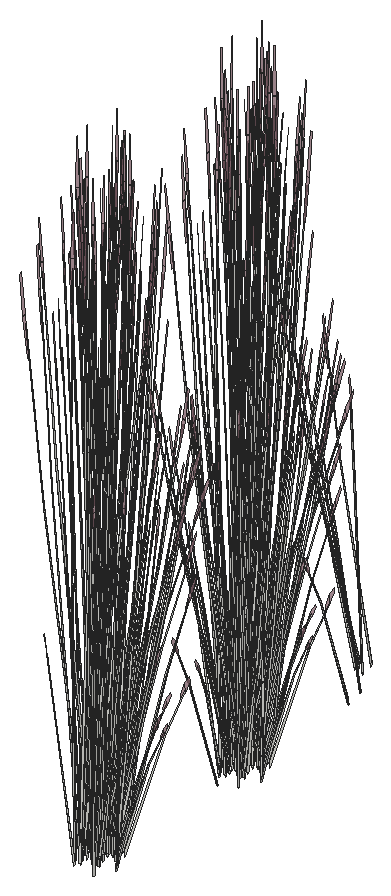
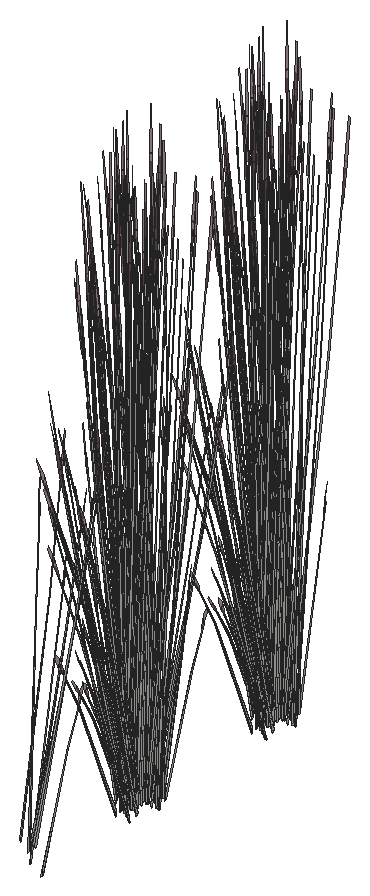
# SketchUp Ruby script. Lengths in inches.
U = 1.inch
M = Sketchup.active_model
def pt(a) = Geom::Point3d.new(a.map { |v| v * U })
def face(e, loops, mat)
  f = e.add_face(loops[0].map { |a| pt(a) })
  loops[1..].each { |l| e.add_face(l.map { |a| pt(a) }).erase! }
  f.material = f.back_material = mat if mat
  f
end
# faces: each face lists its corners as indices into pts; further lists are holes
def faces(e, pts, list, mat = nil) = list.each { |f| face(e, (f[0].is_a?(Array) ? f : [f]).map { |l| l.map { |i| pts[i] } }, mat) }
# xy, xz, yz: faces in a plane at the given z, y or x. An outline is a flat list of corners, or four numbers for a rectangle; further outlines are holes
def ring(l) = l.size == 4 ? [[l[0], l[1]], [l[2], l[1]], [l[2], l[3]], [l[0], l[3]]] : l.each_slice(2).to_a
def flat(e, list, mat, &to3) = list.each { |f| face(e, (f[0].is_a?(Array) ? f : [f]).map { |l| ring(l).map { |u, v| to3.(u, v) } }, mat) }
def xy(e, z, list, mat = nil) = flat(e, list, mat) { |x, y| [x, y, z] }
def xz(e, y, list, mat = nil) = flat(e, list, mat) { |x, z| [x, y, z] }
def yz(e, x, list, mat = nil) = flat(e, list, mat) { |y, z| [x, y, z] }
def lines(e, pts, list) = list.each { |a, b| e.add_line(pt(pts[a]), pt(pts[b])) }
# prism: a flat outline (further loops are holes) pulled along v
def prism(e, loops, v, mat = nil)
  f = face(e, loops, mat); d = Geom::Vector3d.new(v.map { |x| x * U })
  f.pushpull(f.normal.samedirection?(d) ? d.length : -d.length)
end
def box(e, o, s, mat = nil) = prism(e, [[o, [o[0] + s[0], o[1], o[2]], [o[0] + s[0], o[1] + s[1], o[2]], [o[0], o[1] + s[1], o[2]]]], [0, 0, s[2]], mat)
def at(x, y, z, deg = 0) = Geom::Transformation.translation(pt([x, y, z])) * Geom::Transformation.rotation(ORIGIN, Z_AXIS, deg.degrees)
def axes(o, x, y, z) = Geom::Transformation.new([*x, 0, *y, 0, *z, 0, *pt(o).to_a, 1])
def part(name) = M.definitions.add(name)
# library, detail: a bought-in or finely detailed component or shape, given as its bounding box
def library(name, o, s) = part(name).tap { |d| box(d.entities, o, s) }
def detail(e, o, s) = box(e.add_group.entities, o, s)
def put(e, d, t, mat = nil) = e.add_instance(d, t).tap { |i| i.material = mat if mat }
def group(e, t, mat = nil) = e.add_group.tap { |g| g.transformation = t; g.material = mat if mat }.entities
root = M.entities
M.materials.add("LightPink_Translucent").color = [144, 107, 117]
M.materials["LightPink_Translucent"].alpha = 0.75
c1 = part("blade")
p = [[2.15,0.21,22],[0,0.17,0],[0.09,0.45,0],[2.18,0.31,22],[2.29,0.31,22],[0.38,0.45,0],
  [2.48,0.24,33],[2.49,0.24,33],[2.48,0.22,33]]
faces(c1.entities,p,[[0,1,2,3],[4,5,2,3],[6,3,4,7],[8,0,3,6]])
c2 = part("seeds")
p = [[0.3,-0.1,1.38],[-0.01,-0.03,1.59],[-0.01,-0.03,0.03],[0.14,-0.07,-0.07],[0.29,-0.03,3],[0.15,0.01,3.11]]
faces(c2.entities,p,[[0,1,2,3],[1,0,4,5]],"LightPink_Translucent")
c3 = part("blade with seeds")
put(c3.entities,c1,at(0,0,0))
put(c3.entities,c2,axes([2.4,0.25,30.99],[1.5799,-0.05474,1.17369],[-0.12525,1.92788,0.29478],[-0.07173,-0.02425,1.56792]))
put(root,c3,axes([401.49,690.17,2.1],[-0.14494,-0.47823,-0.69835],[0.41752,-0.17223,-0.18329],[-0.01602,-0.16194,1.54149]))
put(root,c3,axes([403.43,688.71,1.49],[-0.05283,-0.03674,1.76342],[-0.13569,-0.41045,-0.26939],[0.09154,-0.11138,0.30037]))
put(root,c3,axes([403.42,689.87,4.98],[0.18436,-0.36797,-0.71045],[0.32306,0.26151,0.08574],[0.11008,-0.13332,1.00501]))
put(root,c3,axes([401.43,688.8,2.375],[-0.22066,-0.46731,0],[0.36918,-0.26061,-0.51607],[0.08408,-0.05936,1.63711]))
put(root,c3,axes([403.41,689.7,4.68],[-0.09067,-0.42583,-0.51099],[0.34336,-0.07449,-0.3958],[0.0984,-0.11438,0.97773]))
put(root,c3,axes([401.92,688.24,2.13],[-0.2439,0.26754,-0.03893],[-0.22348,-0.29302,-0.17649],[-0.01573,-0.08303,0.58215]))
put(root,c3,axes([400.63,690.11,2.02],[0,-0.46636,-0.49651],[0.39487,0,0],[0,-0.10622,1.57504]))
put(root,c3,axes([401.73,688.73,2.02],[0.33032,-0.23318,-0.49651],[0.19744,0.41812,0],[0.07523,-0.05311,1.57504]))
put(root,c3,axes([403.69,689.53,2.59],[-0.12609,-0.01381,1.43002],[-0.12917,-0.37055,-0.30754],[0.1549,-0.10482,0.61141]))
put(root,c3,axes([402.12,689.68,2.06],[0.23773,-0.35053,-0.62353],[0.29532,0.31785,-0.16365],[0.09526,-0.08744,1.37633]))
put(root,c3,axes([403.84,688.85,2.77],[-0.11756,0.2374,1.1486],[-0.10105,-0.31895,0.84392],[0.09709,-0.07992,0.25299]))
put(root,c3,axes([403.67,689.74,4.53],[0.30722,-0.06665,-0.35414],[0.08112,0.381,0.4572],[0.08804,-0.10234,0.87481]))
put(root,c3,axes([401.71,690.3,2.21],[0.17124,-0.42022,-0.44739],[0.35581,0.20224,0.21531],[0,-0.09687,1.43643]))
put(root,c3,axes([401.86,690.09,2.67],[-0.04113,-0.53214,-0.29095],[0.42835,-0.03218,-0.50002],[0.07543,-0.07088,1.59708]))
put(root,c3,axes([400.8,690.12,2.03],[0.24637,-0.29097,-0.30978],[0.24637,0.29097,0.30978],[0,-0.09372,1.38974]))
put(root,c3,axes([401.67,690.65,2.67],[-0.39748,-0.22252,-0.29095],[0.19139,-0.46966,-0.50002],[-0.01249,-0.11531,1.59708]))
put(root,c3,axes([401.81,688.91,2.03],[0.32928,0.11539,-0.30978],[-0.08291,0.40636,0.30978],[0.06638,-0.04686,1.38974]))
put(root,c3,axes([401.92,690.51,2.43],[0.39767,0.22603,0.24065],[-0.19139,0.46966,0.50002],[0,-0.10827,1.60543]))
put(root,c3,axes([401.79,690.19,2.72],[-0.38326,0.02879,0.44739],[-0.03466,-0.47788,-0.21531],[0.06861,-0.04843,1.43643]))
put(root,c3,axes([400.8,690.54,2.48],[0,0.46636,0.49651],[-0.39487,0,0],[0,-0.10622,1.57504]))
put(root,c3,axes([403.57,690.64,4.68],[0.09562,-0.42421,-0.51099],[0.32782,0.1454,-0.3958],[0.13199,-0.0389,0.97773]))
put(root,c3,axes([403.06,688.92,2.375],[0.22066,-0.46731,0],[0.36918,0.26061,-0.51607],[0.08408,0.05936,1.63711]))
put(root,c3,axes([401.78,690.36,2.36],[0.15345,0.52148,0.45755],[-0.43845,0.18134,0.17955],[0.00536,-0.09582,1.58856]))
put(root,c3,axes([403.92,690.76,1.98],[-0.22732,0.05597,1.41583],[-0.03618,-0.44548,0.08104],[0.15921,-0.06743,0.80566]))
put(root,c3,axes([404.34,690.37,2.26],[-0.21881,-0.29821,-0.06488],[0.23965,-0.27324,-0.29416],[0.0679,-0.01924,0.97024]))
put(root,c3,axes([401.7,690.77,2.72],[-0.17124,0.42022,0.44739],[-0.35581,-0.20224,-0.21531],[0,-0.09687,1.43643]))
put(root,c3,axes([402.33,690.41,2.21],[0,-0.53961,0],[0.44133,0,0],[0,0,1.79456]))
put(root,c3,axes([402.87,689.16,2.48],[-0.33032,-0.23318,0.49651],[0.19744,-0.41812,0],[0.07523,0.05311,1.57504]))
put(root,c3,axes([403.51,690.8,4.98],[0.31014,-0.20596,-0.71045],[0.17284,0.42397,0.08574],[0.14985,-0.04816,1.00501]))
put(root,c3,axes([402.12,690.07,2.36],[-0.29264,0.42323,0.45755],[-0.34767,-0.3736,0.17955],[0.07055,-0.04224,1.58856]))
put(root,c3,axes([402.44,690.83,2.3],[-0.32829,-0.4014,-0.06131],[0.32849,-0.40164,0],[-0.01146,-0.01402,1.75571]))
put(root,c3,axes([401.61,689.37,2.47],[-0.10196,0.46348,0.17642],[-0.3731,-0.13116,0.35086],[0.06445,-0.00226,1.60407]))
put(root,c3,axes([401.46,689.74,1.59],[-0.3474,0.18671,1.28929],[-0.11057,-0.53572,0.50096],[0.21332,0.00891,1.46642]))
put(root,c3,axes([402.39,689.89,2.62],[0.06809,-0.4162,0.1448],[0.33266,0.07225,-0.41347],[0.06054,0.04274,1.26744]))
put(root,c3,axes([401.82,690.875,2.36],[0.44609,0.09826,0.45755],[-0.09078,0.55493,0.17955],[-0.06519,-0.05359,1.58856]))
put(root,c3,axes([404.17,690.47,1.49],[-0.01845,-0.0708,1.76342],[0.12793,-0.41416,-0.26939],[0.12905,-0.00596,0.30037]))
put(root,c3,axes([402.25,690,2.72],[-0.21202,-0.39143,0.44739],[0.32115,-0.27564,-0.21531],[0.06861,0.04843,1.43643]))
put(root,c3,axes([401.58,691.76,2.47],[0.37926,-0.12378,0.17642],[0.09365,0.46065,0.35086],[-0.03382,-0.06712,1.60407]))
put(root,c3,axes([402.36,690.02,2.67],[0.35635,-0.30962,-0.29095],[0.23697,0.43749,-0.50002],[0.08792,0.04443,1.59708]))
put(root,c3,axes([403.78,690.84,4.53],[0.29332,0.1301,-0.35414],[-0.08555,0.37955,0.4572],[0.11809,-0.0348,0.87481]))
put(root,c3,axes([403.26,689.2,2.02],[0.33032,0.23318,-0.49651],[-0.19744,0.41812,0],[0.07523,0.05311,1.57504]))
put(root,c3,axes([402.63,690.53,2.21],[0.39487,0,0],[0,0.48281,0],[0,0,1.78407]))
put(root,c3,axes([402.74,689.4,2.47],[-0.37926,0.12378,0.17642],[-0.09365,-0.46065,0.35086],[0.03382,0.06712,1.60407]))
put(root,c3,axes([402.98,690.37,3.875],[-0.14639,0.01056,1.71376],[0.09712,-0.45778,0.13857],[0.20862,0.02831,0.73262]))
put(root,c3,axes([403.17,689.37,2.03],[0.08291,0.40636,-0.30978],[-0.32928,0.11539,0.30978],[0.06638,0.04686,1.38974]))
put(root,c3,axes([402.5,690.28,2.38],[-0.44609,-0.09826,0.49198],[0.09078,-0.55493,0.19306],[0.06519,0.05359,1.70813]))
put(root,c3,axes([402.15,691.65,2.2],[-0.11516,-0.40207,0],[0.32884,-0.1408,0],[0,0,1.54371]))
put(root,c3,axes([402.58,691.6,2.18],[0.37054,-0.15823,-0.19198],[0.1302,0.45581,0.00008],[0.0409,-0.01749,1.73897]))
put(root,c3,axes([402.71,691.79,2.47],[0.10196,-0.46348,0.17642],[0.3731,0.13116,0.35086],[-0.06445,0.00226,1.60407]))
put(root,c3,axes([402.62,690.74,2.21],[0.24637,0.30123,0],[-0.24637,0.30123,0],[0,0,1.69266]))
put(root,c3,axes([403.29,690.6,2.47],[-0.2773,-0.3397,0.17642],[0.27945,-0.32949,0.35086],[-0.03063,0.06937,1.60407]))
put(root,c3,axes([402.78,690.09,2.06],[0.36714,0.07646,-0.62353],[-0.07747,0.47163,-0.16365],[0.10956,0.05715,1.37633]))
put(root,c3,axes([404.4,690.91,2.77],[-0.21807,0.07699,1.1486],[0.10265,-0.31819,0.84392],[0.11568,0.02177,0.25299]))
put(root,c3,axes([402.07,691.83,2.2],[-0.35581,-0.20937,0],[0.17124,-0.43505,0],[0,0,1.62707]))
put(root,c3,axes([402.62,690.38,2.72],[0.17124,-0.42022,0.44739],[0.35581,0.20224,-0.21531],[0,0.09687,1.43643]))
put(root,c3,axes([402.55,690.62,2.29],[0,0.53934,-0.05637],[-0.44133,0,0],[0,0.01695,1.79368]))
put(root,c3,axes([402.58,690.24,2.21],[0.21202,0.39143,-0.44739],[-0.32115,0.27564,0.21531],[0.06861,0.04843,1.43643]))
put(root,c3,axes([404.02,691.9,3.93],[-0.06755,-0.39203,-0.03492],[0.31928,-0.09013,-0.15832],[0.06667,0.02485,0.52218]))
put(root,c3,axes([403.52,690.62,2.48],[0,-0.46636,0.49651],[0.39487,0,0],[0,0.10622,1.57504]))
put(root,c3,axes([402.53,690.97,2.72],[0.38326,-0.02879,0.44739],[0.03466,0.47788,-0.21531],[-0.06861,0.04843,1.43643]))
put(root,c3,axes([402.77,690.48,2.62],[0.32884,-0.136,0.1448],[0.11516,0.38837,-0.41347],[0,0.08547,1.26744]))
put(root,c3,axes([403.99,691.42,2.59],[-0.085,-0.1147,1.43002],[0.1106,-0.37943,-0.30754],[0.17198,0.0514,0.61141]))
put(root,c3,axes([402.47,691.84,2.2],[0.35581,0.20937,0],[-0.17124,0.43505,0],[0,0,1.74954]))
put(root,c3,axes([402.61,692.31,2.19],[-0.21791,-0.46895,-0.05142],[0.36918,-0.26061,0.51607],[-0.09097,0.04465,1.6363]))
put(root,c3,axes([402.53,691.17,2.62],[0.26075,0.2802,0.1448],[-0.2175,0.31612,-0.41347],[-0.06054,0.04274,1.26744]))
put(root,c3,axes([403.21,691.66,4.98],[0.35281,0.01123,-0.71045],[-0.0237,0.47284,0.08574],[0.14947,0.0499,1.00501]))
put(root,c3,axes([402.8125,692.03,2.48],[0.33032,-0.23318,0.49651],[0.19744,0.41812,0],[-0.07523,0.05311,1.57504]))
put(root,c3,axes([402.34,691.67,2.29],[0.15345,0.53576,-0.06012],[-0.43845,0.18773,0],[0.00536,0.01871,1.72173]))
put(root,c3,axes([402.51,692.25,2.03],[-0.32928,-0.11539,-0.30978],[0.08291,-0.40636,0.30978],[-0.06638,0.04686,1.38974]))
put(root,c3,axes([403.78,690.7,2.375],[0.44133,0,0],[0,0.52122,-0.51607],[0,0.11871,1.63711]))
put(root,c3,axes([403.61,690.96,2.2],[-0.44111,-0.00373,-0.04976],[0,-0.52122,0.49943],[-0.01386,0.11865,1.58352]))
put(root,c3,axes([402.65,690.51,2.67],[0.39748,0.22252,-0.29095],[-0.19139,0.46966,-0.50002],[0.01249,0.11531,1.59708]))
put(root,c3,axes([403.42,691.85,4.53],[0.20082,0.29199,-0.35414],[-0.2293,0.2764,0.4572],[0.1165,0.04206,0.87481]))
put(root,c3,axes([403.52,691.04,2.03],[-0.24637,0.29097,-0.30978],[-0.24637,-0.29097,0.30978],[0,0.09372,1.38974]))
put(root,c3,axes([402.46,691.07,2.67],[0.04113,0.53214,-0.29095],[-0.42835,0.03218,-0.50002],[-0.07543,0.07088,1.59708]))
put(root,c3,axes([402.61,690.86,2.21],[-0.17124,0.42022,-0.44739],[-0.35581,-0.20224,0.21531],[0,0.09687,1.43643]))
put(root,c3,axes([402.62,692.06,2.33],[0.44186,0.15158,0.30756],[-0.11054,0.54181,-0.36492],[-0.07313,0.06781,1.64885]))
put(root,c3,axes([402.59,692.43,2.02],[-0.33032,0.23318,-0.49651],[-0.19744,-0.41812,0],[-0.07523,0.05311,1.57504]))
put(root,c3,axes([403.6875,691.05,2.02],[0,0.46636,-0.49651],[-0.39487,0,0],[0,0.10622,1.57504]))
put(root,c3,axes([402.7,691.1,3.875],[-0.1311,-0.08035,1.71376],[0.27131,-0.33708,0.13857],[0.16909,0.15206,0.73262]))
put(root,c3,axes([403.18,692.02,2.77],[-0.19872,-0.13409,1.1486],[0.2566,-0.13625,0.84392],[0.06921,0.11541,0.25299]))
put(root,c3,axes([402.89,692.36,2.375],[0.22066,0.46731,0],[-0.36918,0.26061,-0.51607],[-0.08408,0.05936,1.63711]))
put(root,c3,axes([403.24,692.52,1.49],[0.02571,-0.06733,1.76342],[0.32373,-0.19829,-0.26939],[0.09815,0.10263,0.30037]))
put(root,c3,axes([402.7,690.51,2.84],[-0.00964,-0.43909,1.41272],[0.43635,0.11382,0.59816],[-0.1032,0.24027,1.3335]))
put(root,c3,axes([402.8125,690.99,2.09],[0.12941,0.42699,-0.69212],[-0.37279,0.15378,-0.18165],[0.0143,0.14459,1.52773]))
put(root,c3,axes([402.74,692.2,4.68],[0.34827,-0.11086,-0.51099],[0.06092,0.41983,-0.3958],[0.09354,0.12031,0.97773]))
put(root,c3,axes([403.22,692.63,2.67],[-0.22633,-0.01463,1.0506],[0.14947,-0.31064,0.58006],[0.08941,0.11036,0.8241]))
put(root,c3,axes([402.48,691.875,2.59],[0.00623,-0.15459,1.43002],[0.29764,-0.17268,-0.30754],[0.09188,0.18503,0.61141]))
put(root,c3,axes([401.73,692.5,1.49],[0.05712,-0.02538,1.76342],[0.34359,0.13968,-0.26939],[0.01005,0.15742,0.30037]))
put(root,c3,axes([401.21,692.09,5],[0.25266,0.31335,-0.5672],[-0.2669,0.27442,-0.43934],[-0.03844,0.15921,1.08528]))
put(root,c3,axes([400.9375,692.5625,2.82],[0.32063,-0.08258,0.06507],[0.07371,0.33271,-0.86304],[-0.02033,0.16842,0.7736]))
put(root,c3,axes([401.96,692.4,4.68],[0.34695,0.11691,-0.51099],[-0.11892,0.40083,-0.3958],[0.03181,0.16138,0.97773]))
put(root,c3,axes([402.16,691.57,3.875],[-0.08068,-0.14973,1.71376],[0.3728,-0.12606,0.13857],[0.08426,0.23506,0.73262]))
put(root,c3,axes([401.8,692.64,4.53],[-0.1064,0.35863,-0.35414],[-0.31043,-0.1046,0.4572],[0.02846,0.14439,0.87481]))
put(root,c3,axes([401.5,691.64,3.875],[-0.00864,-0.17899,1.71376],[0.37441,0.11874,0.13857],[-0.02316,0.25508,0.73262]))
put(root,c3,axes([401.84,692.32,4.98],[0.16845,0.3792,-0.71045],[-0.34676,0.21133,0.08574],[0.03939,0.18322,1.00501]))
put(root,c3,axes([402.72,706.15,2.59],[-0.10032,0.0944,1.43002],[-0.30046,-0.16522,-0.30754],[0.05569,-0.20547,0.61141]))
put(root,c3,axes([402.27,706.48,4.98],[-0.16845,-0.3792,-0.71045],[0.34676,-0.21133,0.08574],[-0.03939,-0.18322,1.00501]))
put(root,c3,axes([401.98,705.64,1.49],[-0.0592,0.0168,1.76342],[-0.32738,-0.18913,-0.26939],[0.00549,-0.15776,0.30037]))
put(root,c3,axes([402.97,706.85,4.98],[0.00918,-0.43138,-0.71045],[0.38672,0.02897,0.08574],[0.04081,-0.18275,1.00501]))
put(root,c3,axes([402.3,706.15,4.53],[0.1064,-0.35863,-0.35414],[0.31043,0.1046,0.4572],[-0.02846,-0.14439,0.87481]))
put(root,c3,axes([402.53,706.63,3.875],[-0.06572,0.16029,1.71376],[-0.27569,-0.33172,0.13857],[0.12437,-0.20675,0.73262]))
put(root,c3,axes([402.14,706.4,4.68],[-0.34695,-0.11691,-0.51099],[0.11892,-0.40083,-0.3958],[-0.03181,-0.16138,0.97773]))
put(root,c3,axes([402.35,705.4,2.77],[0.04528,0.27194,1.1486],[-0.25117,-0.15062,0.84392],[0.02703,-0.13924,0.25299]))
put(root,c3,axes([402.89,706.7,4.68],[-0.25266,-0.31335,-0.51099],[0.2669,-0.27442,-0.3958],[0.03844,-0.15921,0.97773]))
put(root,c3,axes([403.13,706.59,4.53],[0.23881,-0.24554,-0.35414],[0.22606,0.28036,0.4572],[0.0344,-0.14245,0.87481]))
put(root,c3,axes([401.49,707.9,2.1],[-0.14494,-0.47823,-0.69835],[0.41752,-0.17223,-0.18329],[-0.01602,-0.16194,1.54149]))
put(root,c3,axes([403.43,706.44,1.49],[-0.05283,-0.03674,1.76342],[-0.13569,-0.41045,-0.26939],[0.09154,-0.11138,0.30037]))
put(root,c3,axes([403.42,707.6,4.98],[0.18436,-0.36797,-0.71045],[0.32306,0.26151,0.08574],[0.11008,-0.13332,1.00501]))
put(root,c3,axes([401.43,706.53,2.375],[-0.22066,-0.46731,0],[0.36918,-0.26061,-0.51607],[0.08408,-0.05936,1.63711]))
put(root,c3,axes([403.41,707.43,4.68],[-0.09067,-0.42583,-0.51099],[0.34336,-0.07449,-0.3958],[0.0984,-0.11438,0.97773]))
put(root,c3,axes([401.92,705.96,2.13],[-0.2439,0.26754,-0.03893],[-0.22348,-0.29302,-0.17649],[-0.01573,-0.08303,0.58215]))
put(root,c3,axes([400.63,707.83,2.02],[0,-0.46636,-0.49651],[0.39487,0,0],[0,-0.10622,1.57504]))
put(root,c3,axes([401.73,706.45,2.02],[0.33032,-0.23318,-0.49651],[0.19744,0.41812,0],[0.07523,-0.05311,1.57504]))
put(root,c3,axes([403.69,707.26,2.59],[-0.12609,-0.01381,1.43002],[-0.12917,-0.37055,-0.30754],[0.1549,-0.10482,0.61141]))
put(root,c3,axes([402.12,707.41,2.06],[0.23773,-0.35053,-0.62353],[0.29532,0.31785,-0.16365],[0.09526,-0.08744,1.37633]))
put(root,c3,axes([403.84,706.58,2.77],[-0.11756,0.2374,1.1486],[-0.10105,-0.31895,0.84392],[0.09709,-0.07992,0.25299]))
put(root,c3,axes([403.67,707.47,4.53],[0.30722,-0.06665,-0.35414],[0.08112,0.381,0.4572],[0.08804,-0.10234,0.87481]))
put(root,c3,axes([401.71,708.02,2.21],[0.17124,-0.42022,-0.44739],[0.35581,0.20224,0.21531],[0,-0.09687,1.43643]))
put(root,c3,axes([401.86,707.82,2.67],[-0.04113,-0.53214,-0.29095],[0.42835,-0.03218,-0.50002],[0.07543,-0.07088,1.59708]))
put(root,c3,axes([400.8,707.84,2.03],[0.24637,-0.29097,-0.30978],[0.24637,0.29097,0.30978],[0,-0.09372,1.38974]))
put(root,c3,axes([401.67,708.375,2.67],[-0.39748,-0.22252,-0.29095],[0.19139,-0.46966,-0.50002],[-0.01249,-0.11531,1.59708]))
put(root,c3,axes([401.81,706.64,2.03],[0.32928,0.11539,-0.30978],[-0.08291,0.40636,0.30978],[0.06638,-0.04686,1.38974]))
put(root,c3,axes([401.92,708.23,2.43],[0.39767,0.22603,0.24065],[-0.19139,0.46966,0.50002],[0,-0.10827,1.60543]))
put(root,c3,axes([401.79,707.92,2.72],[-0.38326,0.02879,0.44739],[-0.03466,-0.47788,-0.21531],[0.06861,-0.04843,1.43643]))
put(root,c3,axes([400.8,708.27,2.48],[0,0.46636,0.49651],[-0.39487,0,0],[0,-0.10622,1.57504]))
put(root,c3,axes([403.57,708.37,4.68],[0.09562,-0.42421,-0.51099],[0.32782,0.1454,-0.3958],[0.13199,-0.0389,0.97773]))
put(root,c3,axes([403.06,706.64,2.375],[0.22066,-0.46731,0],[0.36918,0.26061,-0.51607],[0.08408,0.05936,1.63711]))
put(root,c3,axes([401.78,708.09,2.36],[0.15345,0.52148,0.45755],[-0.43845,0.18134,0.17955],[0.00536,-0.09582,1.58856]))
put(root,c3,axes([403.92,708.49,1.98],[-0.22732,0.05597,1.41583],[-0.03618,-0.44548,0.08104],[0.15921,-0.06743,0.80566]))
put(root,c3,axes([404.34,708.1,2.26],[-0.21881,-0.29821,-0.06488],[0.23965,-0.27324,-0.29416],[0.0679,-0.01924,0.97024]))
put(root,c3,axes([401.7,708.5,2.72],[-0.17124,0.42022,0.44739],[-0.35581,-0.20224,-0.21531],[0,-0.09687,1.43643]))
put(root,c3,axes([402.33,708.14,2.21],[0,-0.53961,0],[0.44133,0,0],[0,0,1.79456]))
put(root,c3,axes([402.87,706.89,2.48],[-0.33032,-0.23318,0.49651],[0.19744,-0.41812,0],[0.07523,0.05311,1.57504]))
put(root,c3,axes([403.51,708.53,4.98],[0.31014,-0.20596,-0.71045],[0.17284,0.42397,0.08574],[0.14985,-0.04816,1.00501]))
put(root,c3,axes([402.12,707.8,2.36],[-0.29264,0.42323,0.45755],[-0.34767,-0.3736,0.17955],[0.07055,-0.04224,1.58856]))
put(root,c3,axes([402.44,708.55,2.3],[-0.32829,-0.4014,-0.06131],[0.32849,-0.40164,0],[-0.01146,-0.01402,1.75571]))
put(root,c3,axes([401.61,707.1,2.47],[-0.10196,0.46348,0.17642],[-0.3731,-0.13116,0.35086],[0.06445,-0.00226,1.60407]))
put(root,c3,axes([401.46,707.47,1.59],[-0.3474,0.18671,1.28929],[-0.11057,-0.53572,0.50096],[0.21332,0.00891,1.46642]))
put(root,c3,axes([402.39,707.61,2.62],[0.06809,-0.4162,0.1448],[0.33266,0.07225,-0.41347],[0.06054,0.04274,1.26744]))
put(root,c3,axes([401.82,708.6,2.36],[0.44609,0.09826,0.45755],[-0.09078,0.55493,0.17955],[-0.06519,-0.05359,1.58856]))
put(root,c3,axes([404.17,708.2,1.49],[-0.01845,-0.0708,1.76342],[0.12793,-0.41416,-0.26939],[0.12905,-0.00596,0.30037]))
put(root,c3,axes([402.25,707.72,2.72],[-0.21202,-0.39143,0.44739],[0.32115,-0.27564,-0.21531],[0.06861,0.04843,1.43643]))
put(root,c3,axes([401.58,709.49,2.47],[0.37926,-0.12378,0.17642],[0.09365,0.46065,0.35086],[-0.03382,-0.06712,1.60407]))
put(root,c3,axes([402.36,707.75,2.67],[0.35635,-0.30962,-0.29095],[0.23697,0.43749,-0.50002],[0.08792,0.04443,1.59708]))
put(root,c3,axes([403.78,708.56,4.53],[0.29332,0.1301,-0.35414],[-0.08555,0.37955,0.4572],[0.11809,-0.0348,0.87481]))
put(root,c3,axes([403.26,706.93,2.02],[0.33032,0.23318,-0.49651],[-0.19744,0.41812,0],[0.07523,0.05311,1.57504]))
put(root,c3,axes([402.63,708.26,2.21],[0.39487,0,0],[0,0.48281,0],[0,0,1.78407]))
put(root,c3,axes([402.74,707.125,2.47],[-0.37926,0.12378,0.17642],[-0.09365,-0.46065,0.35086],[0.03382,0.06712,1.60407]))
put(root,c3,axes([402.98,708.1,3.875],[-0.14639,0.01056,1.71376],[0.09712,-0.45778,0.13857],[0.20862,0.02831,0.73262]))
put(root,c3,axes([403.17,707.1,2.03],[0.08291,0.40636,-0.30978],[-0.32928,0.11539,0.30978],[0.06638,0.04686,1.38974]))
put(root,c3,axes([402.5,708.01,2.38],[-0.44609,-0.09826,0.49198],[0.09078,-0.55493,0.19306],[0.06519,0.05359,1.70813]))
put(root,c3,axes([402.15,709.38,2.2],[-0.11516,-0.40207,0],[0.32884,-0.1408,0],[0,0,1.54371]))
put(root,c3,axes([402.58,709.32,2.18],[0.37054,-0.15823,-0.19198],[0.1302,0.45581,0.00008],[0.0409,-0.01749,1.73897]))
put(root,c3,axes([402.71,709.51,2.47],[0.10196,-0.46348,0.17642],[0.3731,0.13116,0.35086],[-0.06445,0.00226,1.60407]))
put(root,c3,axes([402.62,708.46,2.21],[0.24637,0.30123,0],[-0.24637,0.30123,0],[0,0,1.69266]))
put(root,c3,axes([403.29,708.33,2.47],[-0.2773,-0.3397,0.17642],[0.27945,-0.32949,0.35086],[-0.03063,0.06937,1.60407]))
put(root,c3,axes([402.78,707.82,2.06],[0.36714,0.07646,-0.62353],[-0.07747,0.47163,-0.16365],[0.10956,0.05715,1.37633]))
put(root,c3,axes([404.4,708.64,2.77],[-0.21807,0.07699,1.1486],[0.10265,-0.31819,0.84392],[0.11568,0.02177,0.25299]))
put(root,c3,axes([402.07,709.5625,2.2],[-0.35581,-0.20937,0],[0.17124,-0.43505,0],[0,0,1.62707]))
put(root,c3,axes([402.62,708.11,2.72],[0.17124,-0.42022,0.44739],[0.35581,0.20224,-0.21531],[0,0.09687,1.43643]))
put(root,c3,axes([402.55,708.35,2.29],[0,0.53934,-0.05637],[-0.44133,0,0],[0,0.01695,1.79368]))
put(root,c3,axes([402.58,707.97,2.21],[0.21202,0.39143,-0.44739],[-0.32115,0.27564,0.21531],[0.06861,0.04843,1.43643]))
put(root,c3,axes([404.02,709.625,3.93],[-0.06755,-0.39203,-0.03492],[0.31928,-0.09013,-0.15832],[0.06667,0.02485,0.52218]))
put(root,c3,axes([403.52,708.34,2.48],[0,-0.46636,0.49651],[0.39487,0,0],[0,0.10622,1.57504]))
put(root,c3,axes([402.53,708.69,2.72],[0.38326,-0.02879,0.44739],[0.03466,0.47788,-0.21531],[-0.06861,0.04843,1.43643]))
put(root,c3,axes([402.77,708.21,2.62],[0.32884,-0.136,0.1448],[0.11516,0.38837,-0.41347],[0,0.08547,1.26744]))
put(root,c3,axes([403.99,709.15,2.59],[-0.085,-0.1147,1.43002],[0.1106,-0.37943,-0.30754],[0.17198,0.0514,0.61141]))
put(root,c3,axes([402.47,709.57,2.2],[0.35581,0.20937,0],[-0.17124,0.43505,0],[0,0,1.74954]))
put(root,c3,axes([402.61,710.03,2.19],[-0.21791,-0.46895,-0.05142],[0.36918,-0.26061,0.51607],[-0.09097,0.04465,1.6363]))
put(root,c3,axes([402.53,708.9,2.62],[0.26075,0.2802,0.1448],[-0.2175,0.31612,-0.41347],[-0.06054,0.04274,1.26744]))
put(root,c3,axes([403.21,709.38,4.98],[0.35281,0.01123,-0.71045],[-0.0237,0.47284,0.08574],[0.14947,0.0499,1.00501]))
put(root,c3,axes([402.8125,709.76,2.48],[0.33032,-0.23318,0.49651],[0.19744,0.41812,0],[-0.07523,0.05311,1.57504]))
put(root,c3,axes([402.34,709.39,2.29],[0.15345,0.53576,-0.06012],[-0.43845,0.18773,0],[0.00536,0.01871,1.72173]))
put(root,c3,axes([402.51,709.97,2.03],[-0.32928,-0.11539,-0.30978],[0.08291,-0.40636,0.30978],[-0.06638,0.04686,1.38974]))
put(root,c3,axes([403.78,708.42,2.375],[0.44133,0,0],[0,0.52122,-0.51607],[0,0.11871,1.63711]))
put(root,c3,axes([403.61,708.69,2.2],[-0.44111,-0.00373,-0.04976],[0,-0.52122,0.49943],[-0.01386,0.11865,1.58352]))
put(root,c3,axes([402.65,708.24,2.67],[0.39748,0.22252,-0.29095],[-0.19139,0.46966,-0.50002],[0.01249,0.11531,1.59708]))
put(root,c3,axes([403.42,709.58,4.53],[0.20082,0.29199,-0.35414],[-0.2293,0.2764,0.4572],[0.1165,0.04206,0.87481]))
put(root,c3,axes([403.52,708.77,2.03],[-0.24637,0.29097,-0.30978],[-0.24637,-0.29097,0.30978],[0,0.09372,1.38974]))
put(root,c3,axes([402.46,708.8,2.67],[0.04113,0.53214,-0.29095],[-0.42835,0.03218,-0.50002],[-0.07543,0.07088,1.59708]))
put(root,c3,axes([402.61,708.59,2.21],[-0.17124,0.42022,-0.44739],[-0.35581,-0.20224,0.21531],[0,0.09687,1.43643]))
put(root,c3,axes([402.62,709.79,2.33],[0.44186,0.15158,0.30756],[-0.11054,0.54181,-0.36492],[-0.07313,0.06781,1.64885]))
put(root,c3,axes([402.59,710.16,2.02],[-0.33032,0.23318,-0.49651],[-0.19744,-0.41812,0],[-0.07523,0.05311,1.57504]))
put(root,c3,axes([403.6875,708.78,2.02],[0,0.46636,-0.49651],[-0.39487,0,0],[0,0.10622,1.57504]))
put(root,c3,axes([402.7,708.83,3.875],[-0.1311,-0.08035,1.71376],[0.27131,-0.33708,0.13857],[0.16909,0.15206,0.73262]))
put(root,c3,axes([403.18,709.74,2.77],[-0.19872,-0.13409,1.1486],[0.2566,-0.13625,0.84392],[0.06921,0.11541,0.25299]))
put(root,c3,axes([402.89,710.09,2.375],[0.22066,0.46731,0],[-0.36918,0.26061,-0.51607],[-0.08408,0.05936,1.63711]))
put(root,c3,axes([403.24,710.24,1.49],[0.02571,-0.06733,1.76342],[0.32373,-0.19829,-0.26939],[0.09815,0.10263,0.30037]))
put(root,c3,axes([402.7,708.24,2.84],[-0.00964,-0.43909,1.41272],[0.43635,0.11382,0.59816],[-0.1032,0.24027,1.3335]))
put(root,c3,axes([402.8125,708.71,2.09],[0.12941,0.42699,-0.69212],[-0.37279,0.15378,-0.18165],[0.0143,0.14459,1.52773]))
put(root,c3,axes([402.74,709.93,4.68],[0.34827,-0.11086,-0.51099],[0.06092,0.41983,-0.3958],[0.09354,0.12031,0.97773]))
put(root,c3,axes([403.22,710.36,2.67],[-0.22633,-0.01463,1.0506],[0.14947,-0.31064,0.58006],[0.08941,0.11036,0.8241]))
put(root,c3,axes([402.48,709.6,2.59],[0.00623,-0.15459,1.43002],[0.29764,-0.17268,-0.30754],[0.09188,0.18503,0.61141]))
put(root,c3,axes([401.73,710.23,1.49],[0.05712,-0.02538,1.76342],[0.34359,0.13968,-0.26939],[0.01005,0.15742,0.30037]))
put(root,c3,axes([401.21,709.82,5],[0.25266,0.31335,-0.5672],[-0.2669,0.27442,-0.43934],[-0.03844,0.15921,1.08528]))
put(root,c3,axes([400.9375,710.29,2.82],[0.32063,-0.08258,0.06507],[0.07371,0.33271,-0.86304],[-0.02033,0.16842,0.7736]))
put(root,c3,axes([401.96,710.125,4.68],[0.34695,0.11691,-0.51099],[-0.11892,0.40083,-0.3958],[0.03181,0.16138,0.97773]))
put(root,c3,axes([402.16,709.3,3.875],[-0.08068,-0.14973,1.71376],[0.3728,-0.12606,0.13857],[0.08426,0.23506,0.73262]))
put(root,c3,axes([401.8,710.37,4.53],[-0.1064,0.35863,-0.35414],[-0.31043,-0.1046,0.4572],[0.02846,0.14439,0.87481]))
put(root,c3,axes([401.5,709.37,3.875],[-0.00864,-0.17899,1.71376],[0.37441,0.11874,0.13857],[-0.02316,0.25508,0.73262]))
put(root,c3,axes([401.84,710.05,4.98],[0.16845,0.3792,-0.71045],[-0.34676,0.21133,0.08574],[0.03939,0.18322,1.00501]))
put(root,c3,axes([402.72,722.26,2.59],[-0.10032,0.0944,1.43002],[-0.30046,-0.16522,-0.30754],[0.05569,-0.20547,0.61141]))
put(root,c3,axes([402.27,722.59,4.98],[-0.16845,-0.3792,-0.71045],[0.34676,-0.21133,0.08574],[-0.03939,-0.18322,1.00501]))
put(root,c3,axes([401.98,721.75,1.49],[-0.0592,0.0168,1.76342],[-0.32738,-0.18913,-0.26939],[0.00549,-0.15776,0.30037]))
put(root,c3,axes([402.97,722.96,4.98],[0.00918,-0.43138,-0.71045],[0.38672,0.02897,0.08574],[0.04081,-0.18275,1.00501]))
put(root,c3,axes([402.3,722.27,4.53],[0.1064,-0.35863,-0.35414],[0.31043,0.1046,0.4572],[-0.02846,-0.14439,0.87481]))
put(root,c3,axes([402.53,722.74,3.875],[-0.06572,0.16029,1.71376],[-0.27569,-0.33172,0.13857],[0.12437,-0.20675,0.73262]))
put(root,c3,axes([402.14,722.51,4.68],[-0.34695,-0.11691,-0.51099],[0.11892,-0.40083,-0.3958],[-0.03181,-0.16138,0.97773]))
